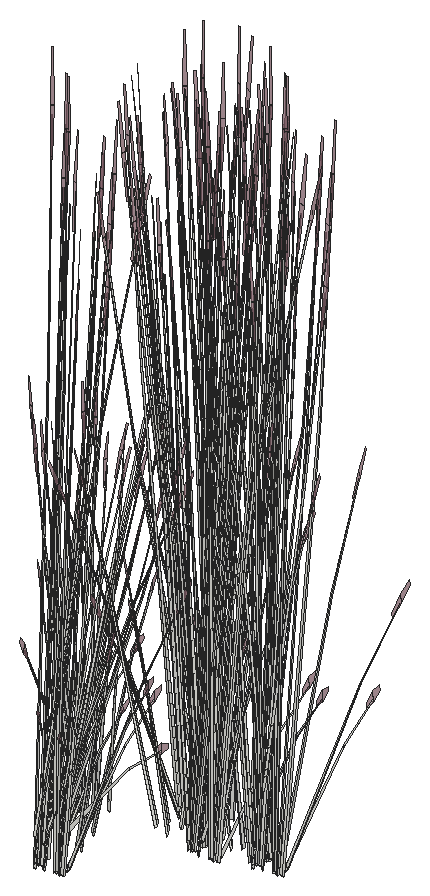
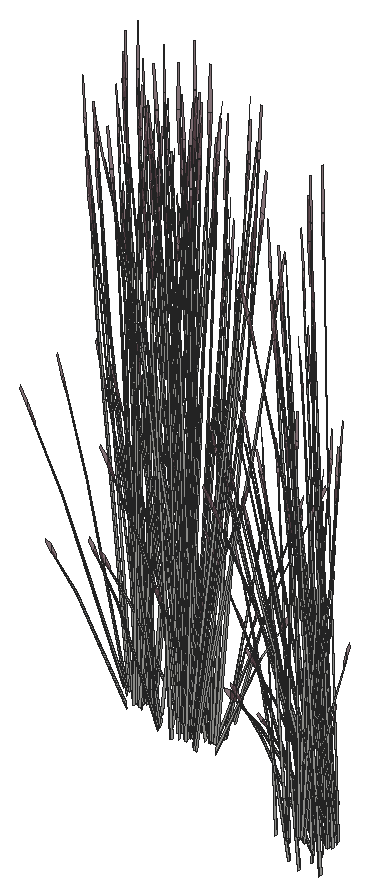
# SketchUp Ruby script. Lengths in inches.
U = 1.inch
M = Sketchup.active_model
def pt(a) = Geom::Point3d.new(a.map { |v| v * U })
def face(e, loops, mat)
  f = e.add_face(loops[0].map { |a| pt(a) })
  loops[1..].each { |l| e.add_face(l.map { |a| pt(a) }).erase! }
  f.material = f.back_material = mat if mat
  f
end
# faces: each face lists its corners as indices into pts; further lists are holes
def faces(e, pts, list, mat = nil) = list.each { |f| face(e, (f[0].is_a?(Array) ? f : [f]).map { |l| l.map { |i| pts[i] } }, mat) }
# xy, xz, yz: faces in a plane at the given z, y or x. An outline is a flat list of corners, or four numbers for a rectangle; further outlines are holes
def ring(l) = l.size == 4 ? [[l[0], l[1]], [l[2], l[1]], [l[2], l[3]], [l[0], l[3]]] : l.each_slice(2).to_a
def flat(e, list, mat, &to3) = list.each { |f| face(e, (f[0].is_a?(Array) ? f : [f]).map { |l| ring(l).map { |u, v| to3.(u, v) } }, mat) }
def xy(e, z, list, mat = nil) = flat(e, list, mat) { |x, y| [x, y, z] }
def xz(e, y, list, mat = nil) = flat(e, list, mat) { |x, z| [x, y, z] }
def yz(e, x, list, mat = nil) = flat(e, list, mat) { |y, z| [x, y, z] }
def lines(e, pts, list) = list.each { |a, b| e.add_line(pt(pts[a]), pt(pts[b])) }
# prism: a flat outline (further loops are holes) pulled along v
def prism(e, loops, v, mat = nil)
  f = face(e, loops, mat); d = Geom::Vector3d.new(v.map { |x| x * U })
  f.pushpull(f.normal.samedirection?(d) ? d.length : -d.length)
end
def box(e, o, s, mat = nil) = prism(e, [[o, [o[0] + s[0], o[1], o[2]], [o[0] + s[0], o[1] + s[1], o[2]], [o[0], o[1] + s[1], o[2]]]], [0, 0, s[2]], mat)
def at(x, y, z, deg = 0) = Geom::Transformation.translation(pt([x, y, z])) * Geom::Transformation.rotation(ORIGIN, Z_AXIS, deg.degrees)
def axes(o, x, y, z) = Geom::Transformation.new([*x, 0, *y, 0, *z, 0, *pt(o).to_a, 1])
def part(name) = M.definitions.add(name)
# library, detail: a bought-in or finely detailed component or shape, given as its bounding box
def library(name, o, s) = part(name).tap { |d| box(d.entities, o, s) }
def detail(e, o, s) = box(e.add_group.entities, o, s)
def put(e, d, t, mat = nil) = e.add_instance(d, t).tap { |i| i.material = mat if mat }
def group(e, t, mat = nil) = e.add_group.tap { |g| g.transformation = t; g.material = mat if mat }.entities
root = M.entities
M.materials.add("LightPink_Translucent").color = [144, 107, 117]
M.materials["LightPink_Translucent"].alpha = 0.75
c1 = part("blade")
p = [[2.15,0.21,22],[0,0.17,0],[0.09,0.45,0],[2.18,0.31,22],[2.29,0.31,22],[0.38,0.45,0],
  [2.48,0.24,33],[2.49,0.24,33],[2.48,0.22,33]]
faces(c1.entities,p,[[0,1,2,3],[4,5,2,3],[6,3,4,7],[8,0,3,6]])
c2 = part("seeds")
p = [[0.3,-0.1,1.38],[-0.01,-0.03,1.59],[-0.01,-0.03,0.03],[0.14,-0.07,-0.07],[0.29,-0.03,3],[0.15,0.01,3.11]]
faces(c2.entities,p,[[0,1,2,3],[1,0,4,5]],"LightPink_Translucent")
c3 = part("blade with seeds")
put(c3.entities,c1,at(0,0,0))
put(c3.entities,c2,axes([2.4,0.25,30.99],[1.5799,-0.05474,1.17369],[-0.12525,1.92788,0.29478],[-0.07173,-0.02425,1.56792]))
put(root,c3,axes([334.47,31.7,50.36],[-0.05884,-0.44587,-0.25709],[0.6128,-0.02696,-0.44182],[0.10791,-0.05939,1.41118]))
put(root,c3,axes([332.95,31.72,49.79],[0.35245,-0.2438,-0.27372],[0.35245,0.2438,0.27372],[0,-0.07853,1.22797]))
put(root,c3,axes([336.06,29.04,50.02],[0.21952,0.44891,-0.05313],[-0.62724,0.1573,0],[0.00767,0.01568,1.52132]))
put(root,c3,axes([323.46,29.02,44.4],[0.24498,-0.3521,0.39531],[0.50902,0.16945,-0.19025],[0,0.08116,1.26923]))
put(root,c3,axes([336.31,29.53,49.79],[-0.47106,-0.09668,-0.27372],[0.11861,-0.34048,0.27372],[-0.09497,0.03926,1.22797]))
put(root,c3,axes([325.87,30.59,46.16],[-0.04566,-0.03421,1.56736],[0.09987,-0.36669,-0.1481],[0.17984,-0.02343,0.27737]))
put(root,c3,axes([332.8125,30.55,49.88],[-0.14565,0.31907,-0.0344],[-0.44829,-0.09815,-0.15595],[-0.06806,-0.05219,0.51438]))
put(root,c3,axes([340.62,29.0625,50.4],[0.24498,-0.3521,0.39531],[0.50902,0.16945,-0.19025],[0,0.08116,1.26923]))
put(root,c3,axes([334.1875,32.16,50.36],[-0.56863,-0.18645,-0.25709],[0.2738,-0.39352,-0.44182],[-0.01787,-0.09662,1.41118]))
put(root,c3,axes([332.91,28.84,50.29],[0.17547,0.03208,1.26356],[0.1131,0.32764,-0.27174],[-0.23835,0.06133,0.54024]))
put(root,c3,axes([332.57,32.01,50.1],[-0.63136,0,0],[0,-0.43672,-0.456],[0,-0.09947,1.44655]))
put(root,c3,axes([338.13,28.23,50.1],[0.63136,0,0],[0,0.43672,-0.456],[0,0.09947,1.44655]))
put(root,c3,axes([323.37,29.22,44.03],[0,0.45191,-0.04981],[-0.63136,0,0],[0,0.0142,1.58489]))
put(root,c3,axes([323.42,28.9,43.95],[0.30332,0.32798,-0.39531],[-0.45944,0.23096,0.19025],[0.09816,0.04058,1.26923]))
put(root,c3,axes([337.88,28.46,49.94],[-0.63105,-0.00312,-0.04397],[0,-0.43672,0.44129],[-0.01983,0.09942,1.3992]))
put(root,c3,axes([332.68,31.23,50.29],[0.09858,0.10879,1.26356],[-0.22716,0.29571,-0.27174],[-0.23325,-0.07068,0.54024]))
put(root,c3,axes([325.47,30.28,45.47],[-0.09664,-0.32847,-0.03085],[0.45676,-0.07551,-0.13989],[0.09538,0.02082,0.4614]))
put(root,c3,axes([340.52,29.26,50.03],[0,0.45191,-0.04981],[-0.63136,0,0],[0,0.0142,1.58489]))
put(root,c3,axes([336.51,28.08,50.36],[0.56863,0.18645,-0.25709],[-0.2738,0.39352,-0.44182],[0.01787,0.09662,1.41118]))
put(root,c3,axes([322.6,33.23,44.29],[-0.14352,0.07909,1.26356],[-0.42983,-0.13843,-0.27174],[0.07968,-0.17216,0.54024]))
put(root,c3,axes([340.57,28.94,49.95],[0.30332,0.32798,-0.39531],[-0.45944,0.23096,0.19025],[0.09816,0.04058,1.26923]))
put(root,c3,axes([324.28,30.27,46.45],[0.02704,-0.39739,-0.10745],[0.51189,0.01086,-0.59638],[0.19715,0.0276,0.90619]))
put(root,c3,axes([334.39,30.71,49.79],[0.47106,0.09668,-0.27372],[-0.11861,0.34048,0.27372],[0.09497,-0.03926,1.22797]))
put(root,c3,axes([338.68,30.62,50.1],[-0.31568,0.39156,0],[-0.52815,-0.21836,-0.456],[-0.12029,-0.04973,1.44655]))
put(root,c3,axes([337.75,28.52,49.79],[-0.35245,0.2438,-0.27372],[-0.35245,-0.2438,0.27372],[0,0.07853,1.22797]))
put(root,c3,axes([324.75,29.21,44.19],[0,-0.39075,0.43871],[0.56491,0,0],[0,0.089,1.3917]))
put(root,c3,axes([336.23,28.54,50.36],[0.05884,0.44587,-0.25709],[-0.6128,0.02696,-0.44182],[-0.10791,0.05939,1.41118]))
put(root,c3,axes([323.68,29.1,44.3125],[0.47043,-0.11396,0.12794],[0.16474,0.32541,-0.36534],[0,0.07162,1.11991]))
put(root,c3,axes([341.9,29.26,50.19],[0,-0.39075,0.43871],[0.56491,0,0],[0,0.089,1.3917]))
put(root,c3,axes([336.45,28.37,49.95],[-0.24498,0.3521,-0.39531],[-0.50902,-0.16945,0.19025],[0,0.08116,1.26923]))
put(root,c3,axes([340.49,29.55,50.4],[0.54829,-0.02412,0.39531],[0.04958,0.40041,-0.19025],[-0.09816,0.04058,1.26923]))
put(root,c3,axes([340.83,29.14,50.3125],[0.47043,-0.11396,0.12794],[0.16474,0.32541,-0.36534],[0,0.07162,1.11991]))
put(root,c3,axes([324.21,30.12,46.46],[-0.28729,-0.24465,0.31292],[0.32804,-0.23159,-0.40398],[0.16667,0.03524,0.77298]))
put(root,c3,axes([340,29.75,49.95],[-0.54829,0.02412,-0.39531],[-0.04958,-0.40041,0.19025],[-0.09816,0.04058,1.26923]))
put(root,c3,axes([325.43,29.89,44.29],[-0.1216,-0.0961,1.26356],[0.15822,-0.31792,-0.27174],[0.24603,0.04307,0.54024]))
put(root,c3,axes([342.58,29.9375,50.29],[-0.1216,-0.0961,1.26356],[0.15822,-0.31792,-0.27174],[0.24603,0.04307,0.54024]))
put(root,c3,axes([322.95,33.82,46.4],[0.01314,-0.36145,-0.62776],[0.55324,0.02428,0.07576],[0.05838,-0.15313,0.88802]))
put(root,c3,axes([323.25,30.24,43.95],[0.50902,0.17543,0],[-0.24498,0.36452,0],[0,0,1.54589]))
put(root,c3,axes([335.86,28.88,49.82],[-0.34009,0.2937,-0.55095],[-0.42248,-0.26632,-0.1446],[-0.13628,0.07327,1.21613]))
put(root,c3,axes([333.06,31.89,50.06],[-0.46965,0.32852,0.27176],[-0.46994,-0.32506,-0.32244],[-0.0164,-0.09329,1.45692]))
put(root,c3,axes([340.4,30.29,49.95],[0.50902,0.17543,0],[-0.24498,0.36452,0],[0,0,1.54589]))
put(root,c3,axes([323.72,33.25,46.17],[-0.00487,-0.07777,1.54581],[-0.41166,-0.22476,-0.24447],[0.06364,-0.13625,0.12397]))
put(root,c3,axes([322.32,33.63,45.43],[-0.09401,0.13431,1.51428],[-0.3944,-0.27795,0.12244],[0.17792,-0.17323,0.64734]))
put(root,c3,axes([323.61,32.97,46.16],[-0.05128,0.02985,1.56736],[-0.5024,-0.1007,-0.1481],[-0.01819,-0.13025,0.27737]))
put(root,c3,axes([336.46,29.38,50.06],[0.63212,0.12701,0.27176],[-0.15814,0.45398,-0.32244],[-0.10462,0.05682,1.45692]))
put(root,c3,axes([324.73,30.04,46.17],[0.10831,-0.00661,1.54581],[0.29709,-0.30358,-0.24447],[0.19266,0.04007,0.12397]))
put(root,c3,axes([336.42,29.68,49.78],[-0.47255,0.19538,-0.43871],[-0.28245,-0.35034,0],[-0.10763,0.0445,1.3917]))
put(root,c3,axes([337.99,28.53,49.78],[0,0.39075,-0.43871],[-0.56491,0,0],[0,0.089,1.3917]))
put(root,c3,axes([340.61,30.67,49.9375],[-0.31175,-0.39292,-0.04544],[0.52815,-0.21836,0.456],[-0.13015,0.03741,1.44584]))
put(root,c3,axes([334.55,32.04,50.15],[0.56891,0.18939,0.21263],[-0.2738,0.39352,0.44182],[0,-0.09071,1.41855]))
put(root,c3,axes([340.5,29.72,50.3125],[0.37303,0.23477,0.12794],[-0.31115,0.26487,-0.36534],[-0.08661,0.03581,1.11991]))
put(root,c3,axes([334.33,32.58,50.16],[0.13383,-0.46302,-0.20702],[0.63453,0.08071,0.45303],[-0.11087,-0.06394,1.38231]))
put(root,c3,axes([322.07,32.6,44.44],[0.06477,0.22786,1.01491],[-0.35932,-0.1262,0.74569],[0.03867,-0.11667,0.22354]))
put(root,c3,axes([322.84,33.7,46.14],[-0.36145,-0.26255,-0.45151],[0.38183,-0.22994,-0.34973],[0.055,-0.1334,0.86392]))
put(root,c3,axes([324.31,30.08,46.4],[0.50473,0.00941,-0.62776],[-0.0339,0.39618,0.07576],[0.21383,0.04181,0.88802]))
put(root,c3,axes([334.37,31.78,50.4],[-0.54829,0.02412,0.39531],[-0.04958,-0.40041,-0.19025],[0.09816,-0.04058,1.26923]))
put(root,c3,axes([332.95,32.07,50.19],[0,0.39075,0.43871],[-0.56491,0,0],[0,-0.089,1.3917]))
put(root,c3,axes([340.89,30.45,50.19],[0.47255,-0.19538,0.43871],[0.28245,0.35034,0],[-0.10763,0.0445,1.3917]))
put(root,c3,axes([323.07,30.09,44.02],[0.21952,0.44891,-0.05313],[-0.62724,0.1573,0],[0.00767,0.01568,1.52132]))
put(root,c3,axes([336.18,30.71,50.1],[0.31568,-0.39156,0],[0.52815,0.21836,-0.456],[0.12029,0.04973,1.44655]))
put(root,c3,axes([340.22,30.14,50.02],[0.21952,0.44891,-0.05313],[-0.62724,0.1573,0],[0.00767,0.01568,1.52132]))
put(root,c3,axes([340.46,30.625,49.79],[-0.47106,-0.09668,-0.27372],[0.11861,-0.34048,0.27372],[-0.09497,0.03926,1.22797]))
put(root,c3,axes([334.29,32.39,49.95],[-0.30332,-0.32798,-0.39531],[0.45944,-0.23096,0.19025],[-0.09816,-0.04058,1.26923]))
put(root,c3,axes([334.35,31.93,50.09],[0.21952,0.43694,0.40429],[-0.62724,0.15194,0.15865],[0.00767,-0.08029,1.40366]))
put(root,c3,axes([336.85,29.625,50.1],[0.31568,0.39156,0],[-0.52815,0.21836,-0.456],[-0.12029,0.04973,1.44655]))
put(root,c3,axes([337.07,29.93,50.29],[0.17547,0.03208,1.26356],[0.1131,0.32764,-0.27174],[-0.23835,0.06133,0.54024]))
put(root,c3,axes([325.13,29.28,44.1],[0.63136,0,0],[0,0.43672,-0.456],[0,0.09947,1.44655]))
put(root,c3,axes([323.21,33.83,46.45],[-0.55492,-0.01936,-0.10745],[0.01517,-0.36657,-0.59638],[0.03855,-0.14118,0.90619]))
put(root,c3,axes([323.17,33.6,46],[0.34164,-0.20573,-0.31292],[0.3234,0.23491,0.40398],[0.04921,-0.11936,0.77298]))
put(root,c3,axes([337.35,29.76,49.32],[0.03679,-0.05641,1.55816],[0.46313,-0.16615,-0.23804],[0.14041,0.08599,0.26541]))
put(root,c3,axes([324.88,29.5,43.94],[-0.63105,-0.00312,-0.04397],[0,-0.43672,0.44129],[-0.01983,0.09942,1.3992]))
put(root,c3,axes([336.74,28.47,49.85],[0.18514,0.35777,-0.61156],[-0.53331,0.12885,-0.16051],[0.02046,0.12115,1.3499]))
put(root,c3,axes([342.29,29.33,50.1],[0.63136,0,0],[0,0.43672,-0.456],[0,0.09947,1.44655]))
put(root,c3,axes([323.52,29.125,44.36],[0.56863,0.18645,-0.25709],[-0.2738,0.39352,-0.44182],[0.01787,0.09662,1.41118]))
put(root,c3,axes([337.42,32.26,49.75],[-0.3252,0.04689,1.25103],[-0.05176,-0.37326,0.07161],[0.22777,-0.0565,0.71188]))
put(root,c3,axes([338.01,31.93,50],[-0.31304,-0.24986,-0.05733],[0.34284,-0.22894,-0.25992],[0.09714,-0.01612,0.85731]))
put(root,c3,axes([333.1,29.71,49.32],[0.06773,0.03904,1.55816],[0.11484,0.36171,-0.23804],[-0.15011,0.07713,0.26541]))
put(root,c3,axes([342.03,29.55,49.94],[-0.63105,-0.00312,-0.04397],[0,-0.43672,0.44129],[-0.01983,0.09942,1.3992]))
put(root,c3,axes([340.67,29.17,50.36],[0.56863,0.18645,-0.25709],[-0.2738,0.39352,-0.44182],[0.01787,0.09662,1.41118]))
put(root,c3,axes([334.24,32.27,50.4],[-0.24498,0.3521,0.39531],[-0.50902,-0.16945,-0.19025],[0,-0.08116,1.26923]))
put(root,c3,axes([324.61,30.25,46],[0.28729,0.24465,-0.31292],[-0.32804,0.23159,0.40398],[0.16667,0.03524,0.77298]))
put(root,c3,axes([324.75,29.57,43.79],[-0.35245,0.2438,-0.27372],[-0.35245,-0.2438,0.27372],[0,0.07853,1.22797]))
put(root,c3,axes([335.14,31.96,49.95],[0,-0.45213,0],[0.63136,0,0],[0,0,1.58567]))
put(root,c3,axes([324.47,30.34,46.18],[-0.02542,0.29714,0.05682],[-0.38391,-0.00815,0.44729],[0.14706,0.03109,0.68204]))
put(root,c3,axes([341.9,29.61,49.79],[-0.35245,0.2438,-0.27372],[-0.35245,-0.2438,0.27372],[0,0.07853,1.22797]))
put(root,c3,axes([323.46,29.42,43.95],[-0.24498,0.3521,-0.39531],[-0.50902,-0.16945,0.19025],[0,0.08116,1.26923]))
put(root,c3,axes([340.38,29.64,50.36],[0.05884,0.44587,-0.25709],[-0.6128,0.02696,-0.44182],[-0.10791,0.05939,1.41118]))
put(root,c3,axes([335.91,30.92,50.19],[-0.47255,-0.19538,0.43871],[0.28245,-0.35034,0],[0.10763,0.0445,1.3917]))
put(root,c3,axes([340.61,29.46,49.95],[-0.24498,0.3521,-0.39531],[-0.50902,-0.16945,0.19025],[0,0.08116,1.26923]))
put(root,c3,axes([324.5,30.25,46.18],[-0.3723,0.25748,0.42415],[-0.32109,-0.27343,0.34973],[0.17467,0.04749,0.87768]))
put(root,c3,axes([337.32,29.85,50.36],[-0.32378,-0.01225,0.92831],[0.21383,-0.26028,0.51254],[0.12791,0.09247,0.72818]))
put(root,c3,axes([334.02,32.51,49.82],[-0.52523,-0.06406,-0.55095],[0.11084,-0.39517,-0.1446],[-0.15674,-0.04788,1.21613]))
put(root,c3,axes([334.84,31.68,50.09],[-0.41865,0.35461,0.40429],[-0.49737,-0.31303,0.15865],[0.10093,-0.03539,1.40366]))
put(root,c3,axes([335.3,32.3125,50.03],[-0.46965,-0.33633,-0.05417],[0.46994,-0.33653,0],[-0.0164,-0.01174,1.55135]))
put(root,c3,axes([334.11,31.09,50.1875],[-0.14586,0.38834,0.15589],[-0.53375,-0.1099,0.31002],[0.0922,-0.00189,1.41735]))
put(root,c3,axes([323.6,33.47,43.32],[-0.07557,-0.03078,1.55816],[-0.19412,-0.34391,-0.23804],[0.13095,-0.09333,0.26541]))
put(root,c3,axes([340.02,29.98,49.82],[-0.34009,0.2937,-0.55095],[-0.42248,-0.26632,-0.1446],[-0.13628,0.07327,1.21613]))
put(root,c3,axes([333.89,31.41,49.41],[-0.49699,0.15644,1.13921],[-0.15819,-0.44887,0.44265],[0.30518,0.00747,1.29573]))
put(root,c3,axes([335.23,31.53,50.3125],[0.09741,-0.34873,0.12794],[0.4759,0.06053,-0.36534],[0.08661,0.03581,1.11991]))
put(root,c3,axes([323.32,30.54,46.46],[-0.07798,-0.31474,0.31292],[0.44579,-0.08311,-0.40398],[0.11974,0.09019,0.77298]))
put(root,c3,axes([324.99,29.58,43.78],[0,0.39075,-0.43871],[-0.56491,0,0],[0,0.089,1.3917]))
put(root,c3,axes([334.41,32.35,50.09],[0.63817,0.08233,0.40429],[-0.12987,0.46497,0.15865],[-0.09326,-0.0449,1.40366]))
put(root,c3,axes([337.77,32.02,49.32],[-0.02639,-0.05932,1.55816],[0.18302,-0.34702,-0.23804],[0.18462,-0.00499,0.26541]))
put(root,c3,axes([323.58,29.62,45.43],[-0.18755,-0.06732,1.51428],[0.38813,-0.28243,0.12244],[0.24191,0.12741,0.64734]))
put(root,c3,axes([340.62,30.47,50.06],[0.63212,0.12701,0.27176],[-0.15814,0.45398,-0.32244],[-0.10462,0.05682,1.45692]))
put(root,c3,axes([340.58,30.78,49.78],[-0.47255,0.19538,-0.43871],[-0.28245,-0.35034,0],[-0.10763,0.0445,1.3917]))
put(root,c3,axes([342.15,29.62,49.78],[0,0.39075,-0.43871],[-0.56491,0,0],[0,0.089,1.3917]))
put(root,c3,axes([336.26,29.22,50.29],[0.00891,-0.12953,1.26356],[0.4258,-0.14469,-0.27174],[0.13144,0.15503,0.54024]))
put(root,c3,axes([332.33,31.96,49.32],[0.0128,0.06158,1.55816],[-0.25814,0.3216,-0.23804],[-0.18336,-0.01621,0.26541]))
put(root,c3,axes([323.62,28.73,45.95],[-0.4363,-0.20303,1.22187],[0.46069,-0.31611,0.5272],[0.14077,0.1905,1.18105]))
put(root,c3,axes([335.03,31.62,50.4],[-0.30332,-0.32798,0.39531],[0.45944,-0.23096,-0.19025],[0.09816,0.04058,1.26923]))
put(root,c3,axes([323.17,33.68,46.18],[0.35954,0.26661,0.42415],[-0.38183,0.22994,0.34973],[0.06632,-0.12508,0.87768]))
put(root,c3,axes([323.31,33.7,46.18],[0.41493,0.01821,0.05682],[-0.01138,0.27493,0.44729],[0.04342,-0.10531,0.68204]))
put(root,c3,axes([333.46,33.12,49.79],[-0.11861,-0.34048,-0.27372],[0.47106,-0.09668,0.27372],[-0.09497,-0.03926,1.22797]))
put(root,c3,axes([324.28,30.39,44.44],[-0.28429,-0.11236,1.01491],[0.36709,-0.11416,0.74569],[0.09901,0.0967,0.22354]))
put(root,c3,axes([323.28,30.71,46.45],[0.30087,-0.33447,-0.10745],[0.43572,0.19269,-0.59638],[0.15146,0.0945,0.90619]))
put(root,c3,axes([323,33.89,46.46],[-0.34164,0.20573,0.31292],[-0.3234,-0.23491,-0.40398],[0.04921,-0.11936,0.77298]))
put(root,c3,axes([334.0625,33.1,50.1875],[0.54257,-0.10371,0.15589],[0.13397,0.38597,0.31002],[-0.04839,-0.05624,1.41735]))
put(root,c3,axes([335.18,31.64,50.36],[0.50979,-0.25942,-0.25709],[0.339,0.36656,-0.44182],[0.12578,0.03723,1.41118]))
put(root,c3,axes([323.6,34.44,46.4],[0.26374,-0.30832,-0.62776],[0.46217,0.21911,0.07576],[0.15748,-0.11171,0.88802]))
put(root,c3,axes([323.59,34.3,46.14],[-0.12971,-0.3568,-0.45151],[0.49122,-0.06241,-0.34973],[0.14077,-0.09583,0.86392]))
put(root,c3,axes([333.33,33.26,49.78],[-0.47255,-0.19538,-0.43871],[0.28245,-0.35034,0],[-0.10763,-0.0445,1.3917]))
put(root,c3,axes([336.47,30.95,49.78],[0.47255,0.19538,-0.43871],[-0.28245,0.35034,0],[0.10763,0.0445,1.3917]))
put(root,c3,axes([335.1875,29.74,49.32],[0.08172,-0.02126,1.55816],[0.49154,0.11703,-0.23804],[0.01437,0.1319,0.26541]))
put(root,c3,axes([335.57,32.0625,49.95],[0.56491,0,0],[0,0.40454,0],[0,0,1.5764]))
put(root,c3,axes([334.61,32.57,50.36],[-0.50979,0.25942,-0.25709],[-0.339,-0.36656,-0.44182],[-0.12578,-0.03723,1.41118]))
put(root,c3,axes([335.73,31.11,50.1875],[-0.54257,0.10371,0.15589],[-0.13397,-0.38597,0.31002],[0.04839,0.05624,1.41735]))
put(root,c3,axes([323.82,34.56,46.45],[-0.46706,-0.21546,-0.10745],[0.26908,-0.31203,-0.59638],[0.13196,-0.10846,0.90619]))
put(root,c3,axes([322.88,30.98,46.16],[0.00149,-0.04731,1.56736],[0.4327,-0.20872,-0.1481],[0.1503,0.0745,0.27737]))
put(root,c3,axes([341,30.72,50.1],[0.31568,0.39156,0],[-0.52815,0.21836,-0.456],[-0.12029,0.04973,1.44655]))
put(root,c3,axes([324.35,30.8,43.32],[0.03679,-0.05641,1.55816],[0.46313,-0.16615,-0.23804],[0.14041,0.08599,0.26541]))
put(root,c3,axes([323.74,29.52,43.85],[0.18514,0.35777,-0.61156],[-0.53331,0.12885,-0.16051],[0.02046,0.12115,1.3499]))
put(root,c3,axes([341.51,30.85,49.32],[0.03679,-0.05641,1.55816],[0.46313,-0.16615,-0.23804],[0.14041,0.08599,0.26541]))
put(root,c3,axes([323.63,30.54,46.14],[0.49824,-0.09289,-0.45151],[0.08716,0.35177,-0.34973],[0.13382,0.10081,0.86392]))
put(root,c3,axes([340.9,29.57,49.85],[0.18514,0.35777,-0.61156],[-0.53331,0.12885,-0.16051],[0.02046,0.12115,1.3499]))
put(root,c3,axes([334.06,29.8,50.49],[0.45869,-0.0692,0.0575],[0.10545,0.27878,-0.76259],[-0.02908,0.14112,0.68355]))
put(root,c3,axes([336.33,31.09,49.79],[0.11861,0.34048,-0.27372],[-0.47106,0.09668,0.27372],[0.09497,0.03926,1.22797]))
put(root,c3,axes([337.25,30.8,49.32],[0.06773,0.03904,1.55816],[0.11484,0.36171,-0.23804],[-0.15011,0.07713,0.26541]))
put(root,c3,axes([322.25,30.59,46.46],[0.15222,-0.30049,0.31292],[0.44409,0.08764,-0.40398],[0.04072,0.12098,0.77298]))
put(root,c3,axes([335.39,31.86,50.1],[-0.63817,-0.08233,0.43472],[0.12987,-0.46497,0.17059],[0.09326,0.0449,1.50931]))
put(root,c3,axes([321.18,33.49,43.78],[0.47255,-0.19538,-0.43871],[0.28245,0.35034,0],[0.10763,-0.0445,1.3917]))
put(root,c3,axes([323.98,34.16,44.29],[-0.18038,-0.01157,1.26356],[-0.18479,-0.31048,-0.27174],[0.22159,-0.08783,0.54024]))
put(root,c3,axes([334.88,33.01,49.95],[-0.16474,-0.33688,0],[0.47043,-0.11798,0],[0,0,1.36402]))
put(root,c3,axes([324.97,34.46,46.16],[-0.06595,-0.00297,1.56736],[-0.27386,-0.31799,-0.1481],[0.10998,-0.10455,0.27737]))
put(root,c3,axes([324.32,30.9,44.36],[-0.32378,-0.01225,0.92831],[0.21383,-0.26028,0.51254],[0.12791,0.09247,0.72818]))
put(root,c3,axes([334.5625,32.6875,50.3125],[-0.09741,0.34873,0.12794],[-0.4759,-0.06053,-0.36534],[-0.08661,-0.03581,1.11991]))
put(root,c3,axes([341.47,30.94,50.36],[-0.32378,-0.01225,0.92831],[0.21383,-0.26028,0.51254],[0.12791,0.09247,0.72818]))
put(root,c3,axes([335.49,32.96,49.93],[0.53009,-0.13258,-0.16963],[0.18627,0.38191,0.00007],[0.05851,-0.01465,1.53656]))
